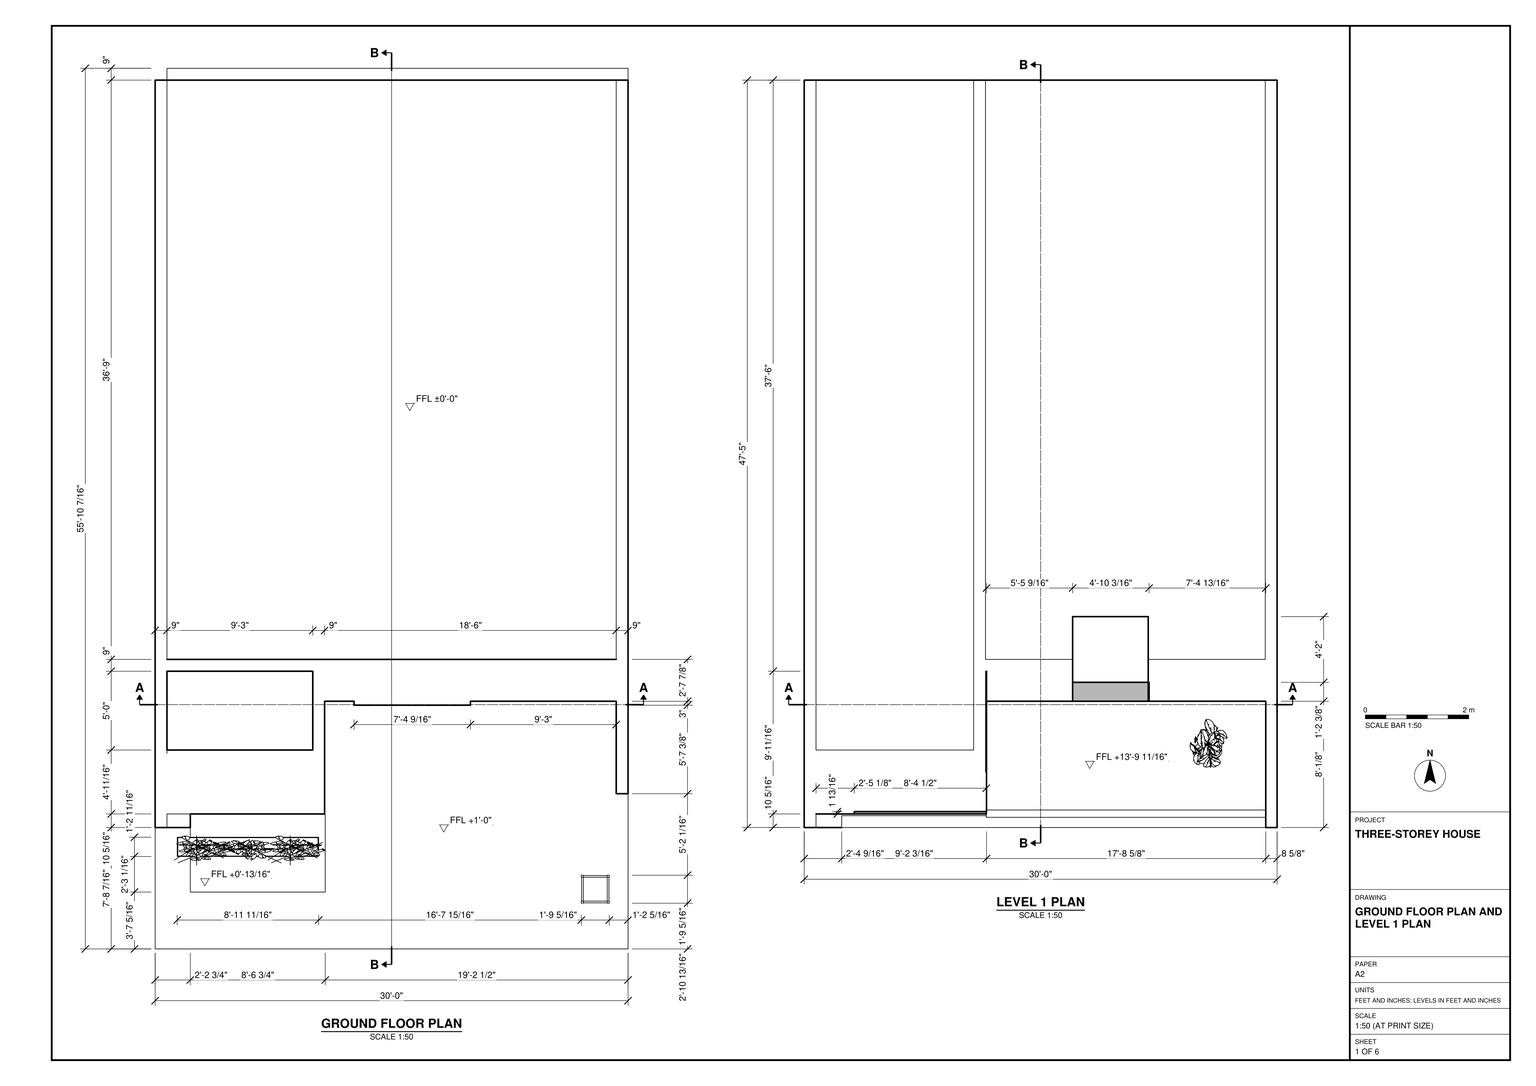
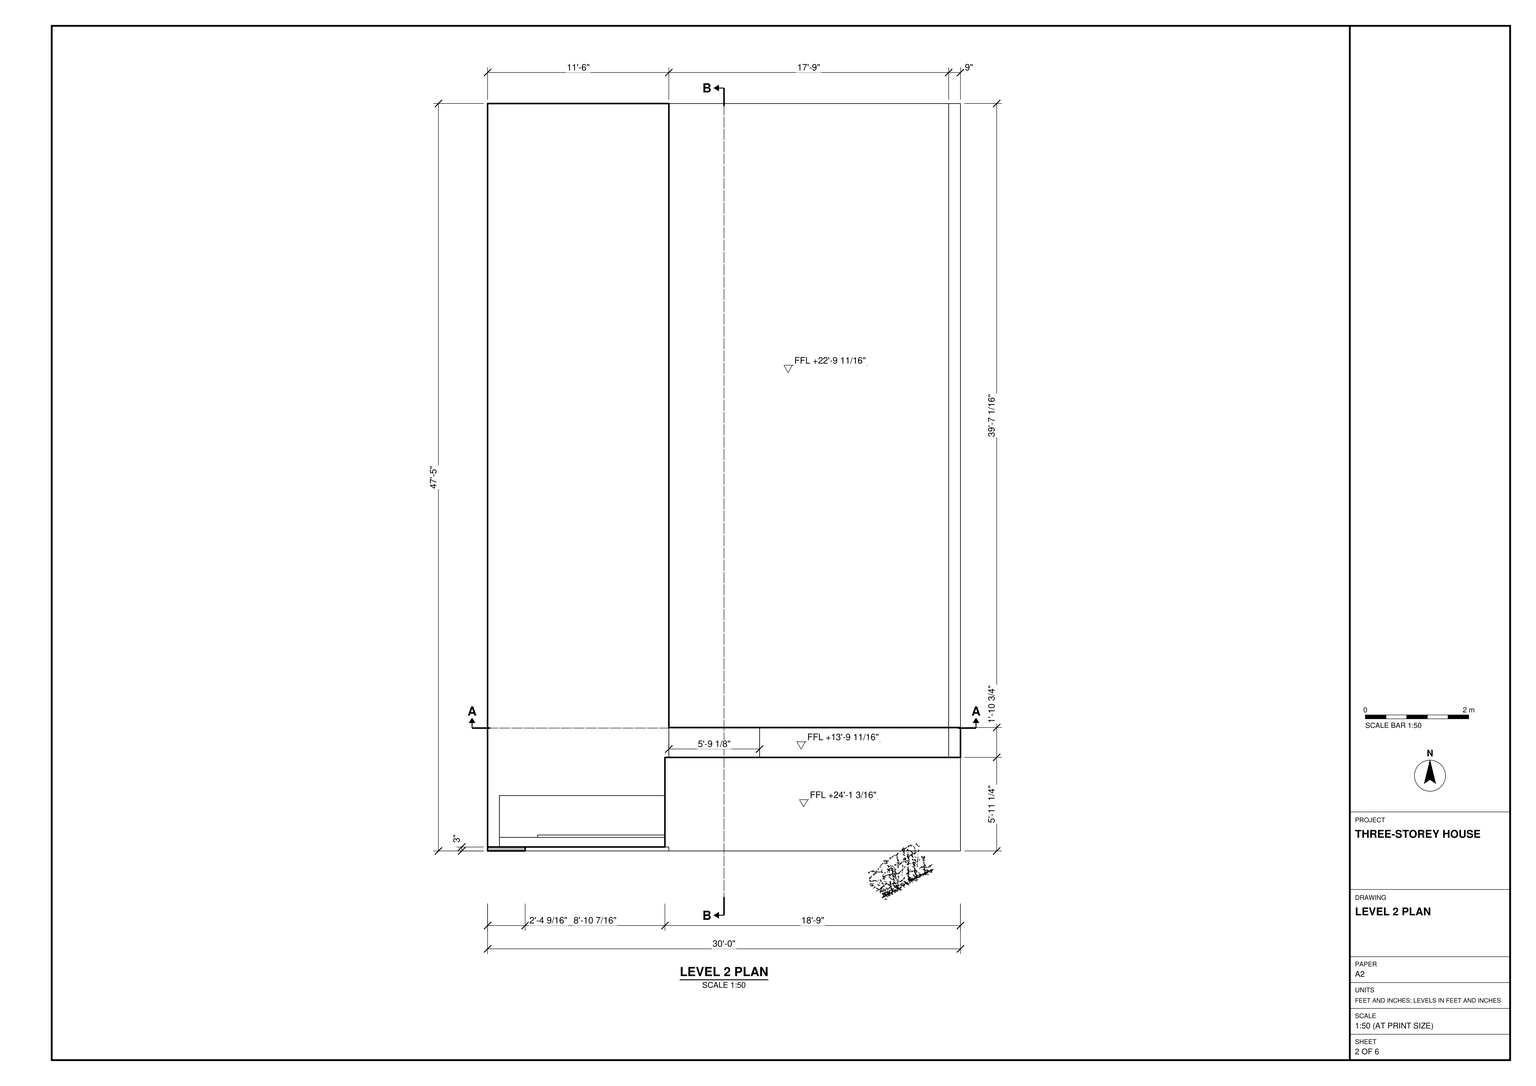
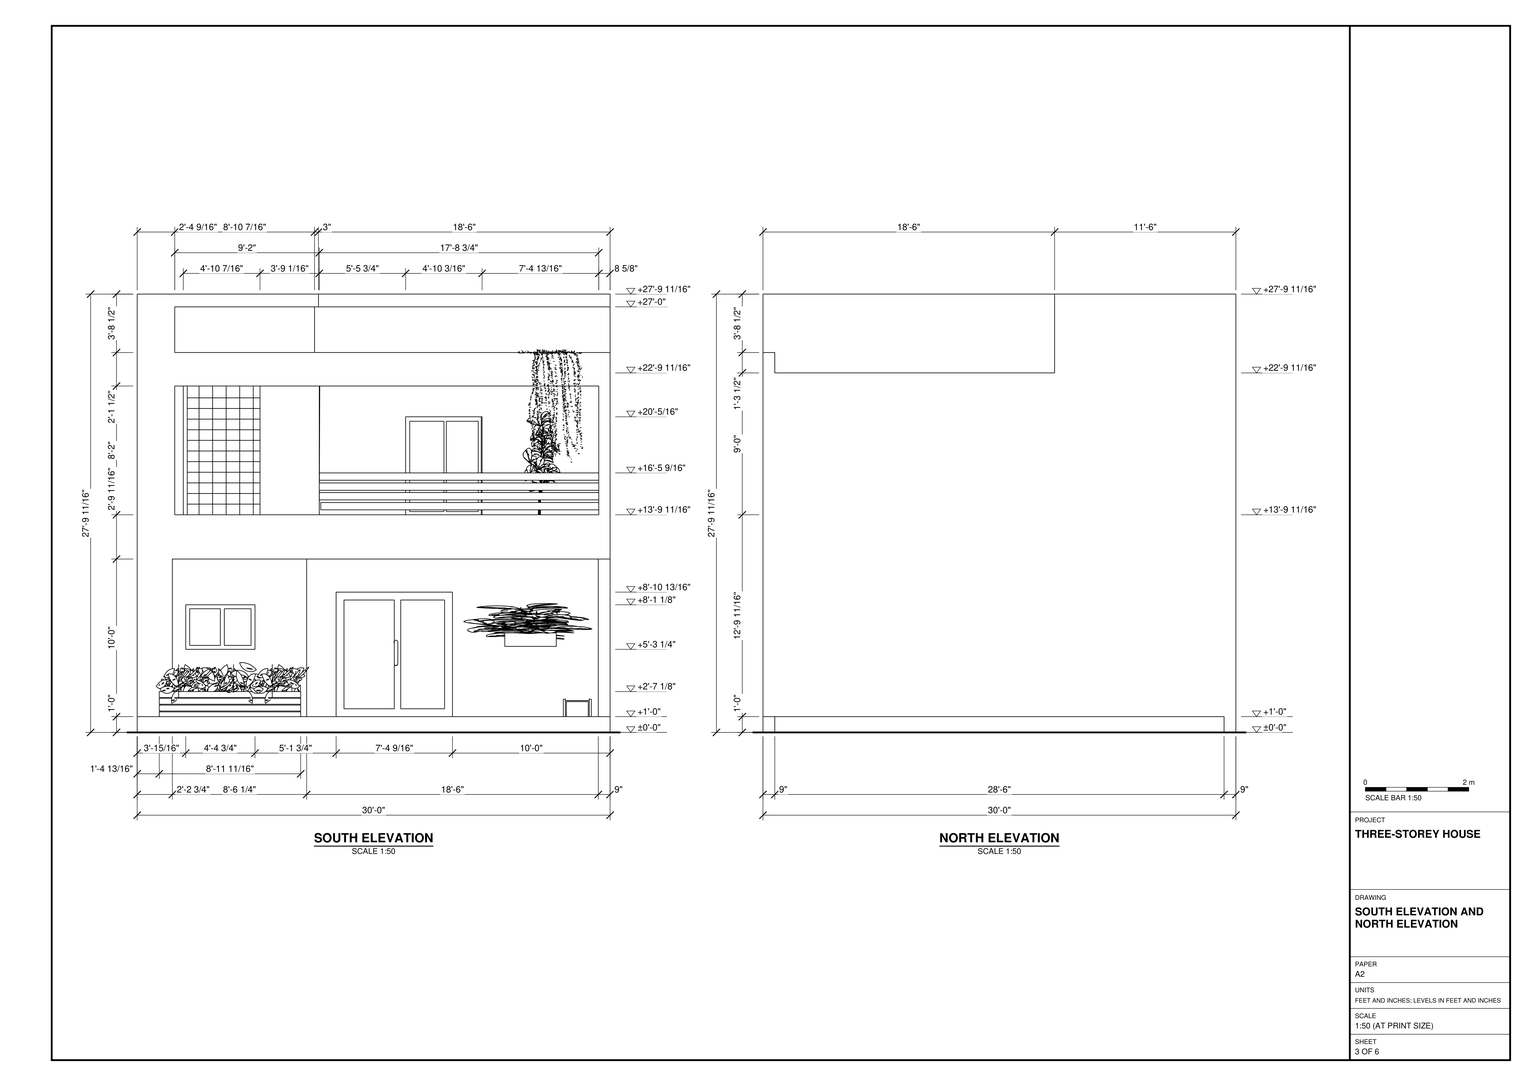
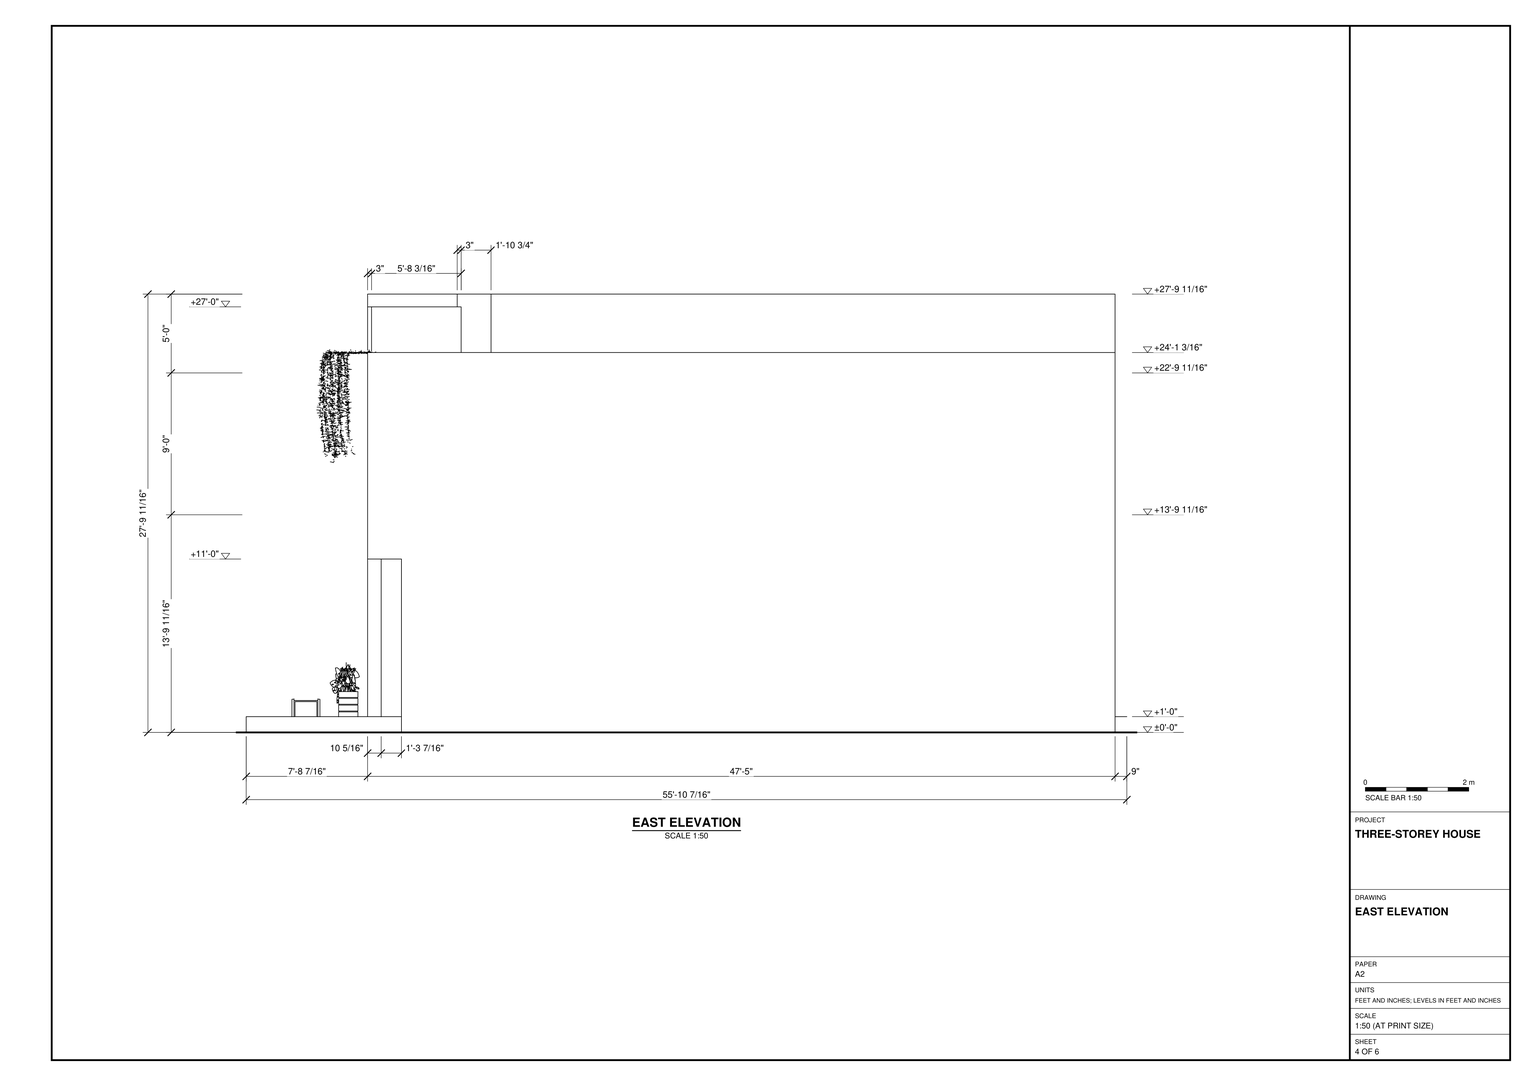
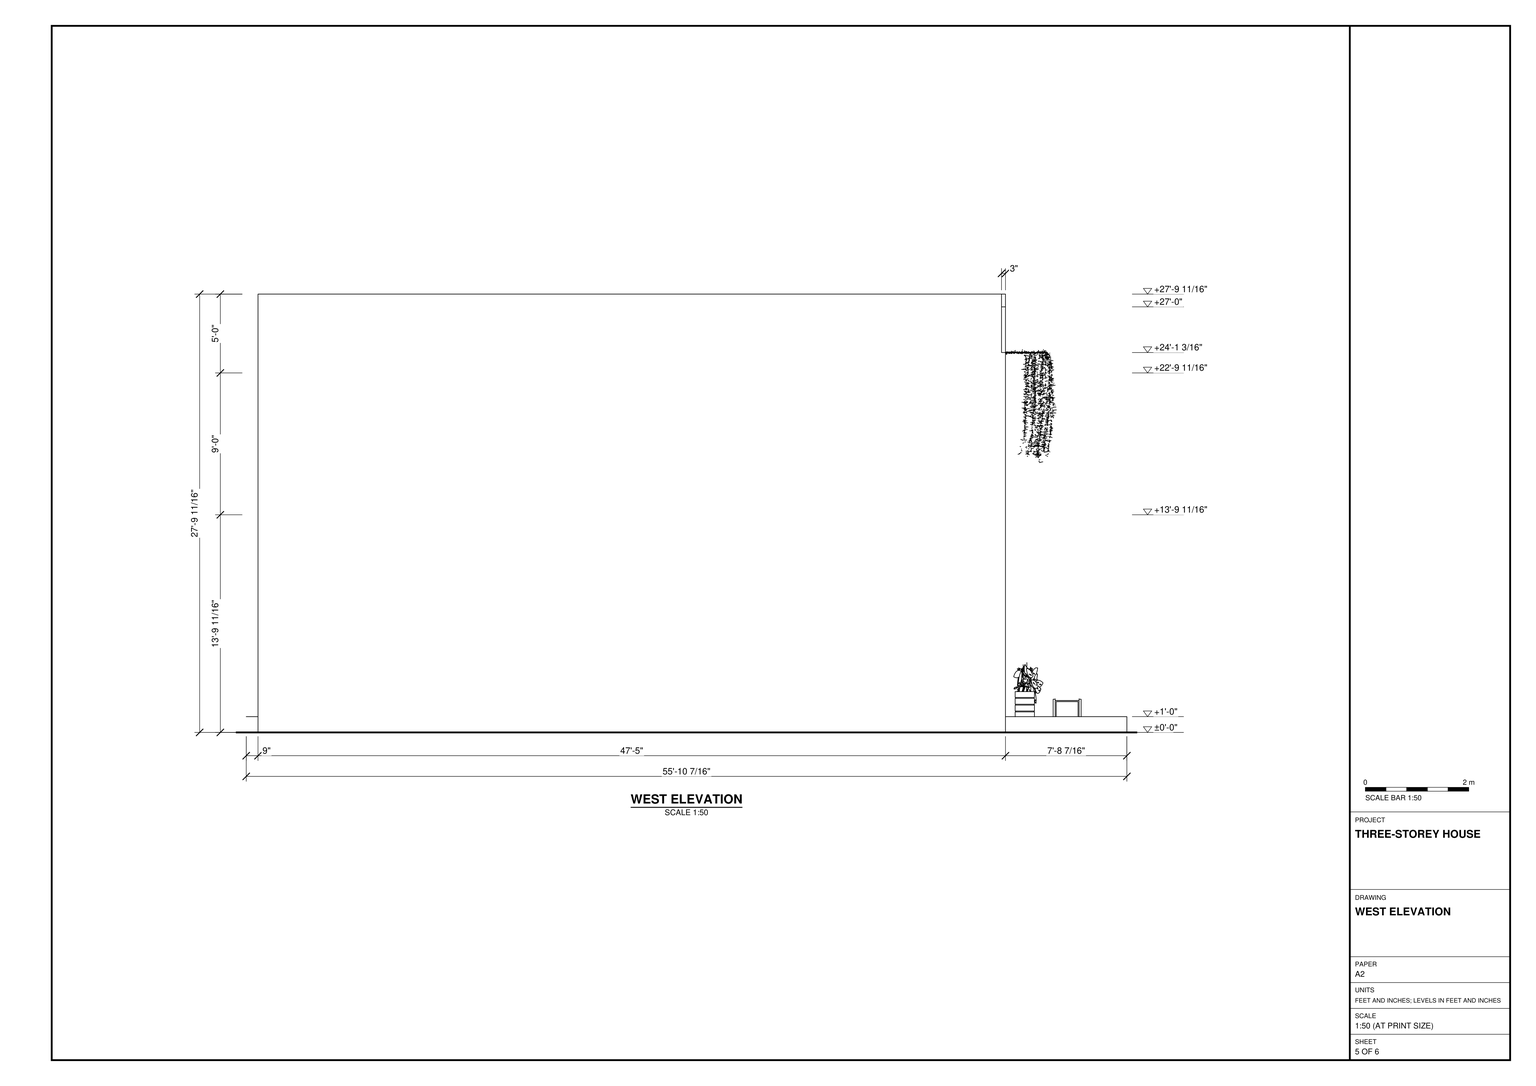
Build the three-storey house shown in task_files/diagram_01.pdf as a SketchUp model. Work in feet and inches. Set the overall width to 30'-0", the front-to-back depth to 55'-10 7/16", and the height to 27'-9 11/16". Use finished floor levels of ±0'-0", +13'-9 11/16", and +22'-9 11/16".

Use the plans to lay out the rectangular base, the stepped ground-floor frontage, the floor slabs, and the walls at their drawn thicknesses, including the 9" perimeter walls. Keep the base extending south beyond the upper floors. On the south elevation, place the paired entrance doors to the right of the smaller window, with the low planted bed beneath the window. Above the entrance, form the recessed balcony with its horizontal railing and paired doors. Model the gridded panel in the adjacent bay. Match the flat roof areas and their changes in height to the upper plan and elevations, including the long horizontal frame above the balcony. Any suitable library components may be used for plants and other loose decor.

Keep walls, slabs, roof elements, and each furniture or joinery piece shown in separate groups or components. Use components for repeated parts. Save one SketchUp model as output_files/three_storey_house_with_a_recessed_south_balcony.skp.

# SketchUp Ruby script. Lengths in inches.
U = 1.inch
M = Sketchup.active_model
def pt(a) = Geom::Point3d.new(a.map { |v| v * U })
def face(e, loops, mat)
  f = e.add_face(loops[0].map { |a| pt(a) })
  loops[1..].each { |l| e.add_face(l.map { |a| pt(a) }).erase! }
  f.material = f.back_material = mat if mat
  f
end
# faces: each face lists its corners as indices into pts; further lists are holes
def faces(e, pts, list, mat = nil) = list.each { |f| face(e, (f[0].is_a?(Array) ? f : [f]).map { |l| l.map { |i| pts[i] } }, mat) }
# xy, xz, yz: faces in a plane at the given z, y or x. An outline is a flat list of corners, or four numbers for a rectangle; further outlines are holes
def ring(l) = l.size == 4 ? [[l[0], l[1]], [l[2], l[1]], [l[2], l[3]], [l[0], l[3]]] : l.each_slice(2).to_a
def flat(e, list, mat, &to3) = list.each { |f| face(e, (f[0].is_a?(Array) ? f : [f]).map { |l| ring(l).map { |u, v| to3.(u, v) } }, mat) }
def xy(e, z, list, mat = nil) = flat(e, list, mat) { |x, y| [x, y, z] }
def xz(e, y, list, mat = nil) = flat(e, list, mat) { |x, z| [x, y, z] }
def yz(e, x, list, mat = nil) = flat(e, list, mat) { |y, z| [x, y, z] }
def lines(e, pts, list) = list.each { |a, b| e.add_line(pt(pts[a]), pt(pts[b])) }
# prism: a flat outline (further loops are holes) pulled along v
def prism(e, loops, v, mat = nil)
  f = face(e, loops, mat); d = Geom::Vector3d.new(v.map { |x| x * U })
  f.pushpull(f.normal.samedirection?(d) ? d.length : -d.length)
end
def box(e, o, s, mat = nil) = prism(e, [[o, [o[0] + s[0], o[1], o[2]], [o[0] + s[0], o[1] + s[1], o[2]], [o[0], o[1] + s[1], o[2]]]], [0, 0, s[2]], mat)
def at(x, y, z, deg = 0) = Geom::Transformation.translation(pt([x, y, z])) * Geom::Transformation.rotation(ORIGIN, Z_AXIS, deg.degrees)
def axes(o, x, y, z) = Geom::Transformation.new([*x, 0, *y, 0, *z, 0, *pt(o).to_a, 1])
def part(name) = M.definitions.add(name)
# library, detail: a bought-in or finely detailed component or shape, given as its bounding box
def library(name, o, s) = part(name).tap { |d| box(d.entities, o, s) }
def detail(e, o, s) = box(e.add_group.entities, o, s)
def put(e, d, t, mat = nil) = e.add_instance(d, t).tap { |i| i.material = mat if mat }
def group(e, t, mat = nil) = e.add_group.tap { |g| g.transformation = t; g.material = mat if mat }.entities
root = M.entities
M.materials.add("!长灌木1").color = [90, 107, 61]
M.materials.add("Brick_14_1K").color = [201, 199, 193]
M.materials.add("Glass_Mirror_01").color = [185, 185, 185]
M.materials.add("Glass_Sky Reflection_01").color = [126, 138, 183]
M.materials["Glass_Sky Reflection_01"].alpha = 0.25
M.materials.add("Material20").color = [184, 138, 65]
M.materials.add("Material48").color = [126, 124, 110]
M.materials.add("Material~1").color = [39, 255, 54]
M.materials.add("Metal_32_1K").color = [117, 124, 125]
M.materials.add("Plywood_08_1K").color = [202, 166, 113]
M.materials.add("ThomThom - Buttons2").color = [40, 40, 43]
M.materials.add("ThomThom - Waistcoat2").color = [127, 127, 126]
M.materials.add("Wood_Floor_01_1K").color = [146, 111, 76]
M.materials.add("Wood_Planks_01_1K").color = [69, 67, 63]
M.materials.add("Wood_Veneer_15_1K").color = [103, 69, 45]
M.materials.add("[Cladding_Siding_Tan]").color = [83, 83, 83]
M.materials.add("avelã ou canyon").color = [164, 137, 111]
c1 = part("Wooden planter box")
xy(c1.entities,0,[[13.83,7.95,28.79,88.09]],"[Cladding_Siding_Tan]")
xy(c1.entities,22.64,[[13.83,7.95,28.79,88.09]],"[Cladding_Siding_Tan]")
xz(c1.entities,7.95,[[13.83,3.9375,28.79,4.53],[13.83,8.46,28.79,9.06],[13.83,12.99,28.79,13.58],[13.83,17.52,28.79,18.11],[13.83,22.05,28.79,22.64]],"[Cladding_Siding_Tan]")
xz(c1.entities,88.09,[[13.83,3.9375,28.79,4.53],[13.83,8.46,28.79,9.06],[13.83,12.99,28.79,13.58],[13.83,17.52,28.79,18.11],[13.83,22.05,28.79,22.64]],"[Cladding_Siding_Tan]")
yz(c1.entities,13.83,[[7.95,3.9375,88.09,4.53],[7.95,8.46,88.09,9.06],[7.95,12.99,88.09,13.58],[7.95,17.52,88.09,18.11],[7.95,22.05,88.09,22.64]],"[Cladding_Siding_Tan]")
yz(c1.entities,28.79,[[7.95,3.9375,88.09,4.53],[7.95,8.46,88.09,9.06],[7.95,12.99,88.09,13.58],[7.95,17.52,88.09,18.11],[7.95,22.05,88.09,22.64]],"[Cladding_Siding_Tan]")
g1 = group(c1.entities,at(13.4375,7.55,0))
prism(g1,[[[15.75,80.93,22.64],[15.75,0,22.64],[0,0,22.64],[0,80.93,22.64]],[[0.39,80.53,22.64],[0.39,0.39,22.64],[15.35,0.39,22.64],[15.35,80.53,22.64]]],[0,0,3.9375],"avelã ou canyon")
prism(g1,[[[15.75,80.93,9.06],[15.75,0,9.06],[0,0,9.06],[0,80.93,9.06]],[[0.39,80.53,9.06],[0.39,0.39,9.06],[15.35,0.39,9.06],[15.35,80.53,9.06]]],[0,0,3.9375],"avelã ou canyon")
prism(g1,[[[15.75,80.93,13.58],[15.75,0,13.58],[0,0,13.58],[0,80.93,13.58]],[[0.39,80.53,13.58],[0.39,0.39,13.58],[15.35,0.39,13.58],[15.35,80.53,13.58]]],[0,0,3.9375],"avelã ou canyon")
prism(g1,[[[15.75,80.93,0],[15.75,0,0],[0,0,0],[0,80.93,0]],[[0.39,80.53,0],[0.39,0.39,0],[15.35,0.39,0],[15.35,80.53,0]]],[0,0,3.9375],"avelã ou canyon")
prism(g1,[[[15.75,80.93,4.53],[15.75,0,4.53],[0,0,4.53],[0,80.93,4.53]],[[0.39,80.53,4.53],[0.39,0.39,4.53],[15.35,0.39,4.53],[15.35,80.53,4.53]]],[0,0,3.9375],"avelã ou canyon")
prism(g1,[[[15.75,80.93,18.11],[15.75,0,18.11],[0,0,18.11],[0,80.93,18.11]],[[0.39,80.53,18.11],[0.39,0.39,18.11],[15.35,0.39,18.11],[15.35,80.53,18.11]]],[0,0,3.9375],"avelã ou canyon")
c2 = library("Bush\#1",[-12.92,-38.23,78.84],[28.51,16.75,15.79])
c3 = library("Bush",[-8.21,-45.67,79.34],[21.65,20.96,14.54])
c4 = library("Group6\#1",[8874.76,-5589.78,-33.6],[50.13,38.07,87.13])
c5 = part("组\#1")
xy(c5.entities,0,[[0,0,2.36,2.36],[29.92,0,32.28,2.36],[0,29.92,2.36,32.28],[29.92,29.92,32.28,32.28]],"Material48")
xy(c5.entities,1.57,[[2.36,0.39,2.36,2.36,0.39,2.36,0.39,29.92,2.36,29.92,2.36,31.89,29.92,31.89,29.92,29.92,31.89,29.92,31.89,2.36,29.92,2.36,29.92,0.39]],"Material48")
xy(c5.entities,2.76,[[3.54,0.39,28.74,1.57],[0.39,3.54,1.57,28.74],[30.71,3.54,31.89,28.74],[3.54,30.71,28.74,31.89]],"Material20")
xy(c5.entities,20.08,[[3.54,0.39,28.74,1.57],[0.39,3.54,1.57,28.74],[30.71,3.54,31.89,28.74],[3.54,30.71,28.74,31.89]],"Material20")
xy(c5.entities,21.0625,[[2.36,2.36,29.92,29.92]],"!长灌木1")
xy(c5.entities,21.26,[[2.36,0.39,29.92,2.36],[0.39,2.36,2.36,29.92],[29.92,2.36,31.89,29.92],[2.36,29.92,29.92,31.89]],"Material20")
xy(c5.entities,21.38,[[2.36,2.36,29.92,29.92]],"!长灌木1")
xy(c5.entities,22.83,[[0,0,2.36,2.36],[29.92,0,32.28,2.36],[0,29.92,2.36,32.28],[29.92,29.92,32.28,32.28]],"Material20")
xz(c5.entities,0,[[0,0,2.36,22.83],[29.92,0,32.28,22.83]],"Material20")
xz(c5.entities,0.39,[[[2.36,1.57,29.92,21.26],[3.54,2.76,28.74,20.08]]],"Material20")
xz(c5.entities,1.57,[[3.54,2.76,28.74,20.08]],"Material20")
xz(c5.entities,2.36,[[2.36,21.0625,29.92,21.38],[2.36,21.26,29.92,23.43]],"!长灌木1")
xz(c5.entities,2.36,[[0,0,0,22.83,2.36,22.83,2.36,21.26,0.39,21.26,0.39,1.57,2.36,1.57,2.36,0],[29.92,0,29.92,1.57,31.89,1.57,31.89,21.26,29.92,21.26,29.92,22.83,32.28,22.83,32.28,0]],"Material20")
xz(c5.entities,3.54,[[0.39,2.76,1.57,20.08],[30.71,2.76,31.89,20.08]],"Material20")
xz(c5.entities,28.74,[[0.39,2.76,1.57,20.08],[30.71,2.76,31.89,20.08]],"Material20")
xz(c5.entities,29.92,[[2.36,21.0625,29.92,21.38],[2.36,21.26,29.92,23.43]],"!长灌木1")
xz(c5.entities,29.92,[[0,0,2.36,0,2.36,1.57,0.39,1.57,0.39,22.83,0,22.83],[29.92,0,32.28,0,32.28,22.83,31.89,22.83,31.89,1.57,29.92,1.57],[0.39,21.26,2.36,22.83],[29.92,21.26,31.89,22.83]],"Material20")
xz(c5.entities,30.71,[[3.54,2.76,28.74,20.08]],"Material20")
xz(c5.entities,31.89,[[[2.36,1.57,29.92,21.26],[3.54,2.76,28.74,20.08]]],"Material20")
xz(c5.entities,32.28,[[0,0,2.36,22.83],[29.92,0,32.28,22.83]],"Material20")
yz(c5.entities,0,[[0,0,2.36,22.83],[29.92,0,32.28,22.83]],"Material20")
yz(c5.entities,0.39,[[[2.36,1.57,29.92,21.26],[3.54,2.76,28.74,20.08]]],"Material20")
yz(c5.entities,1.57,[[3.54,2.76,28.74,20.08]],"Material20")
yz(c5.entities,2.36,[[0,0,2.36,0,2.36,1.57,0.39,1.57,0.39,22.83,0,22.83]])
yz(c5.entities,2.36,[[2.36,21.0625,29.92,21.38],[2.36,21.26,29.92,23.43]],"!长灌木1")
yz(c5.entities,2.36,[[29.92,0,32.28,0,32.28,22.83,29.92,22.83,29.92,21.26,31.89,21.26,31.89,1.57,29.92,1.57],[0.39,21.26,2.36,22.83]],"Material20")
yz(c5.entities,3.54,[[0.39,2.76,1.57,20.08],[30.71,2.76,31.89,20.08]],"Material20")
yz(c5.entities,28.74,[[0.39,2.76,1.57,20.08],[30.71,2.76,31.89,20.08]],"Material20")
yz(c5.entities,29.92,[[2.36,21.0625,29.92,21.38],[2.36,21.26,29.92,23.43]],"!长灌木1")
yz(c5.entities,29.92,[[0,0,0,22.83,2.36,22.83,2.36,21.26,0.39,21.26,0.39,1.57,2.36,1.57,2.36,0],[29.92,0,29.92,1.57,31.89,1.57,31.89,21.26,29.92,21.26,29.92,22.83,32.28,22.83,32.28,0]],"Material20")
yz(c5.entities,30.71,[[3.54,2.76,28.74,20.08]],"Material20")
yz(c5.entities,31.89,[[[2.36,1.57,29.92,21.26],[3.54,2.76,28.74,20.08]]],"Material20")
yz(c5.entities,32.28,[[0,0,2.36,22.83],[29.92,0,32.28,22.83]],"Material20")
c6 = part("组\#2")
put(c6.entities,c5,at(24.1,23.99,0))
c7 = library("Group38\#2",[14.01,28.44,-23.43],[18.58,18.32,38.89])
xy(root,-12,[[0,0,0,92.43,9,92.43,9,102.77,129,102.77,129,142.43,351,142.43,351,118.19,360,118.19,360,0],[[0,92.43,9,92.43,9,102.77,129,102.77,129,188.58,151.43,188.58,151.43,185.58,240,185.58,240,188.58,351,188.58,351,118.19,360,118.19,360,661.43,351,661.43,351,220.43,9,220.43,9,661.43,0,661.43],[9,151.43,120,211.43]],[9,151.43,120,211.43],[9,220.43,351,661.43]])
xy(root,-11.2,[[26.77,43.3,129.49,102.77],[9,92.43,26.77,102.77]])
xy(root,0,[[0,0,360,0,360,118.19,351,118.19,351,188.58,240,188.58,240,185.58,151.43,185.58,151.43,188.58,129,188.58,129,102.77,129.49,102.77,129.49,43.3,26.77,43.3,26.77,92.43,0,92.43],[9,661.43,360,670.43]])
xy(root,51.26,[[36.94,102.77,89.67,188.58]])
xy(root,53.5,[[279.82,154.66,319.02,188.58]],"ThomThom - Waistcoat2")
xy(root,58.53,[[284.25,159.09,314.59,184.15]],"Wood_Veneer_15_1K")
xy(root,63.77,[[[279.82,154.66,319.02,188.58],[284.25,159.09,314.59,184.15]]],"Plywood_08_1K")
xy(root,85.15,[[36.94,102.77,89.67,188.58]])
xy(root,94.8,[[151.43,185.58,240,188.58]])
xy(root,120,[[26.77,92.43,129,102.77],[129,92.43,351,188.58],[351,92.43,360,118.19],[9,151.43,120,211.43]])
xy(root,153.7,[[28.58,92.43,351.38,101.43],[138.6,101.43,351.38,104.56],[38.09,102.77,138.6,104.56],[138,134.6,138.6,211.43],[204.34,188.58,261.9,253]])
xy(root,153.7,[[138.6,104.56,351.38,188.58]],"Glass_Mirror_01")
xy(root,228.29,[[204.34,188.58,261.9,253]],"ThomThom - Waistcoat2")
xy(root,251.7,[[138.98,92.43,138.98,188.58,207.1,188.58,207.1,186.4,351.38,186.4,351.38,92.43],[9,102.77,9,134.6,138.6,134.6,138.6,104.56,38.09,104.56,38.09,102.77],[38.09,102.77,138.6,104.56],[207.1,186.4,351,188.58],[351,186.4,351.38,188.58],
  [138.98,188.58,207.1,211.43]])
xy(root,261.7,[[138,163.64,207.1,186.4],[138,186.4,351,661.43]])
xy(root,277.21,[[28.58,92.43,138,95.43],[138,92.43,360,92.43,360,160.64,351,160.64,351,163.64,135,163.64,135,95.43,138,95.43],[351,160.64,360,163.64],[351,163.64,360,186.4],[351,186.4,360,661.43]])
xy(root,311.98,[[28.58,92.43,138,95.43],[135,95.43,138,163.64],[138,160.64,207.1,163.64],[207.1,160.64,360,163.64]])
xy(root,321.7,[[0,92.43,138,92.43,138,160.64,360,160.64,360,186.4,138,186.4,138,661.43,0,661.43]])
xz(root,0,[[0,-12,360,0]])
xz(root,43.3,[[26.77,-11.2,129.49,0]])
xz(root,92.43,[[[0,0,26.77,0,26.77,120,360,120,360,277.21,28.58,277.21,28.58,311.98,138,311.98,138,321.7,0,321.7],[28.58,153.7,351.38,251.7]]])
xz(root,95.43,[[0,277.21,28.58,311.98],[28.58,277.21,135,311.98]],"ThomThom - Waistcoat2")
xz(root,102.77,[[129,-11.2,129.49,0]])
xz(root,102.77,[[9,-12,129,-11.2],[[26.77,-11.2,129,120],[36.94,51.26,89.67,85.15]]],"Brick_14_1K")
xz(root,102.77,[[39.94,54.26,63.3,82.15],[66.3,54.26,86.67,82.15]],"Glass_Mirror_01")
xz(root,102.77,[[38.09,153.7,47.09,161.79],[47.09,153.7,57.41,161.79],[57.41,153.7,67.72,161.79],[67.72,153.7,78.04,161.79],[78.04,153.7,88.35,161.79],
  [88.35,153.7,93.51,161.79],[38.09,161.79,47.09,169.88],[47.09,161.79,57.41,169.88],[57.41,161.79,67.72,169.88],[67.72,161.79,78.04,169.88],
  [78.04,161.79,88.35,169.88],[88.35,161.79,93.51,169.88],[38.09,169.88,47.09,177.97],[47.09,169.88,57.41,177.97],[57.41,169.88,67.72,177.97],
  [67.72,169.88,78.04,177.97],[78.04,169.88,88.35,177.97],[88.35,169.88,93.51,177.97],[38.09,177.97,47.09,186.06],[47.09,177.97,57.41,186.06],
  [57.41,177.97,67.72,186.06],[67.72,177.97,78.04,186.06],[78.04,177.97,88.35,186.06],[88.35,177.97,93.51,186.06],[38.09,186.06,47.09,194.16],
  [47.09,186.06,57.41,194.16],[57.41,186.06,67.72,194.16],[67.72,186.06,78.04,194.16],[78.04,186.06,88.35,194.16],[88.35,186.06,93.51,194.16],
  [38.09,194.16,47.09,202.25],[47.09,194.16,57.41,202.25],[57.41,194.16,67.72,202.25],[67.72,194.16,78.04,202.25],[78.04,194.16,88.35,202.25],
  [88.35,194.16,93.51,202.25],[38.09,202.25,47.09,210.34],[47.09,202.25,57.41,210.34],[57.41,202.25,67.72,210.34],[67.72,202.25,78.04,210.34],
  [78.04,202.25,88.35,210.34],[88.35,202.25,93.51,210.34],[38.09,210.34,47.09,218.43],[47.09,210.34,57.41,218.43],[57.41,210.34,67.72,218.43],
  [67.72,210.34,78.04,218.43],[78.04,210.34,88.35,218.43],[88.35,210.34,93.51,218.43],[38.09,218.43,47.09,226.52],[47.09,218.43,57.41,226.52],
  [57.41,218.43,67.72,226.52],[67.72,218.43,78.04,226.52],[78.04,218.43,88.35,226.52],[88.35,218.43,93.51,226.52],[38.09,226.52,47.09,234.61],
  [47.09,226.52,57.41,234.61],[57.41,226.52,67.72,234.61],[67.72,226.52,78.04,234.61],[78.04,226.52,88.35,234.61],[88.35,226.52,93.51,234.61],
  [38.09,234.61,47.09,242.7],[47.09,234.61,57.41,242.7],[57.41,234.61,67.72,242.7],[67.72,234.61,78.04,242.7],[78.04,234.61,88.35,242.7],
  [88.35,234.61,93.51,242.7],[38.09,242.7,47.09,251.7],[47.09,242.7,57.41,251.7],[57.41,242.7,67.72,251.7],[67.72,242.7,78.04,251.7],
  [78.04,242.7,88.35,251.7],[88.35,242.7,93.51,251.7]],"Glass_Sky Reflection_01")
xz(root,102.77,[[[36.94,51.26,89.67,85.15],[39.94,54.26,63.3,82.15],[66.3,54.26,86.67,82.15]],[35.09,153.7,38.09,251.7]],"Metal_32_1K")
xz(root,102.77,[[9,153.7,35.09,251.7],[93.51,153.7,138.6,251.7]],"ThomThom - Waistcoat2")
xz(root,104.56,[[38.09,153.7,138.6,251.7],[138.6,153.7,138.61,155.56,138.61,157.58,138.98,251.7,138.6,251.7]],"ThomThom - Waistcoat2")
xz(root,118.19,[[351,-12,360,0],[351,0,360,120]])
xz(root,151.43,[[9,-12,120,120]])
xz(root,154.66,[[279.82,53.5,319.02,63.77]],"Plywood_08_1K")
xz(root,159.09,[[284.25,58.53,314.59,63.77]],"ThomThom - Waistcoat2")
xz(root,160.64,[[138,311.98,360,321.7]])
xz(root,163.64,[[138,261.7,207.1,277.21]])
xz(root,163.64,[[135,277.21,360,311.98]],"ThomThom - Waistcoat2")
xz(root,169.96,[[196.91,55.24,196.52,55.29,196.16,55.4375,195.86,55.67,195.71,55.86,195.71,57.59,195.86,57.77,196.16,58.01,196.52,58.16,196.91,58.21,197.29,58.16,197.65,58.01,197.96,57.77,198.19,57.46,198.34,57.11,198.39,56.72,198.34,56.34,198.19,55.98,197.96,55.67,197.65,55.4375,197.29,55.29]],"Wood_Floor_01_1K")
xz(root,170.0625,[[196.91,38.8125,197.29,38.86,197.65,39.01,197.96,39.25,198.19,39.55,198.34,39.91,198.39,40.3,198.38,40.39,198.34,40.1,198.19,39.74,197.96,39.43,197.65,39.2,197.29,39.05,196.91,39,196.52,39.05,196.16,39.2,195.86,39.43,195.71,39.62,195.71,39.43,195.86,39.25,196.16,39.01,196.52,38.86]],"Wood_Floor_01_1K")
xz(root,184.15,[[284.25,58.53,314.59,63.77]],"Wood_Veneer_15_1K")
xz(root,185.58,[[151.43,-12,240,0]])
xz(root,185.58,[[157.43,6,195.71,6,195.71,55.86,195.62,55.98,195.47,56.34,195.42,56.72,195.47,57.11,195.62,57.46,195.71,57.59,195.71,88.8,157.43,88.8],[200.62,6,234,88.8],[195.71,55.86,195.71,57.59,195.62,57.46,195.47,57.11,195.42,56.72,195.47,56.34,195.62,55.98]],"Glass_Mirror_01")
xz(root,185.58,[[[151.43,0,240,94.8],[157.43,6,157.43,88.8,195.71,88.8,195.71,57.59,195.86,57.77,196.16,58.01,196.52,58.16,196.91,58.21,197.29,58.16,197.65,58.01,197.96,57.77,198.19,57.46,198.34,57.11,198.39,56.72,198.34,56.34,198.19,55.98,197.96,55.67,197.65,55.4375,197.29,55.29,196.91,55.24,196.52,55.29,196.16,55.4375,195.86,55.67,195.71,55.86,195.71,41.16,195.86,41.35,196.16,41.58,196.52,41.73,196.91,41.78,197.29,41.73,197.65,41.58,197.96,41.35,198.19,41.04,198.34,40.68,198.39,40.3,198.34,39.91,198.19,39.55,197.96,39.25,197.65,39.01,197.29,38.86,196.91,38.8125,196.52,38.86,196.16,39.01,195.86,39.25,195.71,39.43,195.71,6],[200.62,6,234,88.8]]],"Wood_Floor_01_1K")
xz(root,186.4,[[207.1,251.7,351,261.7],[138,261.7,138,321.7,360,321.7,360,277.21,351,277.21,351,261.7]])
xz(root,188.58,[[129,-12,151.43,0],[240,-12,351,0],[36.94,51.26,89.67,85.15]])
xz(root,188.58,[[[129,0,151.43,0,151.43,94.8,240,94.8,240,0,351,0,351,120,129,120],[279.82,53.5,319.02,63.77]],[138.6,153.7,204.34,153.7,204.34,228.29,261.9,228.29,261.9,153.7,351.38,153.7,351.38,251.7,138.98,251.7]],"ThomThom - Waistcoat2")
xz(root,211.43,[[9,-12,120,120]])
xz(root,220.43,[[9,-12,351,120]])
xz(root,253,[[204.34,153.7,261.9,228.29]],"ThomThom - Waistcoat2")
xz(root,661.43,[[0,-12,0,321.7,138,321.7,138,261.7,351,261.7,351,277.21,360,277.21,360,0,9,0,9,-12],[9,-12,351,0],[351,-12,360,0]])
yz(root,0,[[0,-12,92.43,0],[92.43,-12,92.43,277.21,95.43,277.21,95.43,321.7,661.43,321.7,661.43,-12],[92.43,277.21,95.43,311.98],[92.43,311.98,95.43,321.7]])
yz(root,9,[[92.43,-12,102.77,-11.2],[151.43,-12,211.43,120]])
yz(root,26.77,[[43.3,-11.2,102.77,-11.2,102.77,120,92.43,120,92.43,0,43.3,0]])
yz(root,28.58,[[92.43,277.21,95.43,311.98]])
yz(root,36.94,[[102.77,51.26,188.58,85.15]])
yz(root,38.09,[[102.77,153.7,104.56,161.79],[102.77,161.79,104.56,169.88],[102.77,169.88,104.56,177.97],[102.77,177.97,104.56,186.06],[102.77,186.06,104.56,194.16],
  [102.77,194.16,104.56,202.25],[102.77,202.25,104.56,210.34],[102.77,210.34,104.56,218.43],[102.77,218.43,104.56,226.52],[102.77,226.52,104.56,234.61],
  [102.77,234.61,104.56,242.7],[102.77,242.7,104.56,251.7]])
yz(root,89.67,[[102.77,51.26,188.58,85.15]])
yz(root,120,[[151.43,-12,211.43,120]])
yz(root,129,[[142.43,-12,188.58,0]])
yz(root,129,[[102.77,-12,142.43,0],[102.77,0,188.58,120]],"ThomThom - Waistcoat2")
yz(root,129.49,[[43.3,-11.2,102.77,0]])
yz(root,135,[[95.43,277.21,163.64,311.98]])
yz(root,138,[[163.64,261.7,186.4,277.21],[186.4,261.7,661.43,321.7],[92.43,311.98,160.64,321.7]])
yz(root,138.6,[[102.77,172.36,102.28,172.43,101.6,172.71,101.03,173.15,100.59,173.73,100.31,174.4,100.21,175.12,100.31,175.84,100.59,176.51,101.03,177.09,101.6,177.53,102.28,177.81,102.77,177.875],[104.56,172.84,104.56,177.4,104.97,177.09,105.41,176.51,105.6875,175.84,105.78,175.12,105.6875,174.4,105.41,173.73,104.97,173.15]])
yz(root,138.6,[[102.77,153.7,102.77,172.36,103,172.33,103.72,172.43,104.39,172.71,104.56,172.84,104.56,153.7],[103,172.33,102.77,172.36,102.77,177.875,103,177.9,103.72,177.81,104.39,177.53,104.56,177.4,104.56,172.84,104.39,172.71,103.72,172.43],[104.56,177.4,104.39,177.53,103.72,177.81,103,177.9,102.77,177.875,102.77,251.7,104.56,251.7]],"ThomThom - Waistcoat2")
yz(root,138.61,[[104.56,155.56,104.56,157.58,104.3,157.54,104.06,157.44,103.85,157.28,103.6875,157.07,103.58,156.83,103.55,156.57,103.58,156.31,103.6875,156.0625,103.85,155.85,104.06,155.69,104.3,155.59]])
yz(root,138.61,[[104.56,155.56,104.82,155.59,105.07,155.69,105.27,155.85,105.44,156.0625,105.54,156.31,105.57,156.57,105.54,156.83,105.44,157.07,105.27,157.28,105.07,157.44,104.82,157.54,104.56,157.58]],"ThomThom - Waistcoat2")
yz(root,138.66,[[103,165.04,102.28,165.13,101.6,165.41,101.03,165.85,100.59,166.43,100.31,167.1,100.21,167.82,100.31,168.54,100.59,169.21,101.03,169.79,101.6,170.23,102.28,170.51,103,170.61,103.72,170.51,104.39,170.23,104.97,169.79,105.41,169.21,105.6875,168.54,105.78,167.82,105.6875,167.1,105.41,166.43,104.97,165.85,104.39,165.41,103.72,165.13],[103,179.98,102.28,180.08,101.6,180.36,101.03,180.8,100.59,181.375,100.31,182.05,100.21,182.77,100.31,183.49,100.59,184.16,101.03,184.74,101.6,185.18,102.28,185.46,103,185.55,103.72,185.46,104.39,185.18,104.97,184.74,105.41,184.16,105.6875,183.49,105.78,182.77,105.6875,182.05,105.41,181.375,104.97,180.8,104.39,180.36,103.72,180.08]])
yz(root,139.74,[[103,157.45,102.28,157.54,101.6,157.82,101.03,158.26,100.59,158.84,100.31,159.51,100.21,160.23,100.31,160.95,100.59,161.625,101.03,162.2,101.6,162.64,102.28,162.92,103,163.02,103.72,162.92,104.39,162.64,104.97,162.2,105.41,161.625,105.6875,160.95,105.78,160.23,105.6875,159.51,105.41,158.84,104.97,158.26,104.39,157.82,103.72,157.54]])
yz(root,151.43,[[185.58,-12,188.58,0],[185.58,0,188.58,94.8]])
yz(root,195.71,[[170.0625,39.43,185.58,41.16],[167.2,39.62,167.2,57.59,169.96,57.59,169.96,55.86,168.93,55.86,168.93,41.35,170.0625,41.35,170.0625,39.62],[169.96,55.86,185.58,57.59]],"Wood_Planks_01_1K")
yz(root,204.34,[[188.58,153.7,253,228.29]],"ThomThom - Waistcoat2")
yz(root,240,[[185.58,-12,188.58,0],[185.58,0,188.58,94.8]])
yz(root,261.9,[[188.58,153.7,253,228.29]],"ThomThom - Waistcoat2")
yz(root,279.82,[[154.66,53.5,188.58,63.77]],"Plywood_08_1K")
yz(root,284.25,[[159.09,58.53,184.15,63.77]],"ThomThom - Waistcoat2")
yz(root,314.59,[[159.09,58.53,184.15,63.77]],"Wood_Veneer_15_1K")
yz(root,319.02,[[154.66,53.5,188.58,63.77]],"ThomThom - Waistcoat2")
yz(root,351,[[118.19,-12,142.43,0],[142.43,-12,188.58,0],[118.19,0,188.58,120],[186.4,251.7,211.43,261.7],[186.4,261.7,661.43,277.21]])
yz(root,351.38,[[[92.43,153.7,188.58,251.7],[103,179.98,103.72,180.08,104.39,180.36,104.97,180.8,105.41,181.375,105.6875,182.05,105.78,182.77,105.6875,183.49,105.41,184.16,104.97,184.74,104.39,185.18,103.72,185.46,103,185.55,102.28,185.46,101.6,185.18,101.03,184.74,100.59,184.16,100.31,183.49,100.21,182.77,100.31,182.05,100.59,181.375,101.03,180.8,101.6,180.36,102.28,180.08],[103,157.45,103.72,157.54,104.39,157.82,104.97,158.26,105.41,158.84,105.6875,159.51,105.78,160.23,105.6875,160.95,105.41,161.625,104.97,162.2,104.39,162.64,103.72,162.92,103,163.02,102.28,162.92,101.6,162.64,101.03,162.2,100.59,161.625,100.31,160.95,100.21,160.23,100.31,159.51,100.59,158.84,101.03,158.26,101.6,157.82,102.28,157.54],[103,165.04,103.72,165.13,104.39,165.41,104.97,165.85,105.41,166.43,105.6875,167.1,105.78,167.82,105.6875,168.54,105.41,169.21,104.97,169.79,104.39,170.23,103.72,170.51,103,170.61,102.28,170.51,101.6,170.23,101.03,169.79,100.59,169.21,100.31,168.54,100.21,167.82,100.31,167.1,100.59,166.43,101.03,165.85,101.6,165.41,102.28,165.13],[103,172.33,103.72,172.43,104.39,172.71,104.97,173.15,105.41,173.73,105.6875,174.4,105.78,175.12,105.6875,175.84,105.41,176.51,104.97,177.09,104.39,177.53,103.72,177.81,103,177.9,102.28,177.81,101.6,177.53,101.03,177.09,100.59,176.51,100.31,175.84,100.21,175.12,100.31,174.4,100.59,173.73,101.03,173.15,101.6,172.71,102.28,172.43]]])
yz(root,360,[[0,-12,118.19,0],[118.19,-12,661.43,-12,661.43,277.21,92.43,277.21,92.43,120,118.19,120],[163.64,277.21,186.4,277.21,186.4,321.7,160.64,321.7,160.64,311.98,163.64,311.98]])
# 35 loose lines left out
p = [[196.52,185.58,38.86],[196.91,185.58,38.8125],[196.91,170.0625,38.8125],[196.52,170.0625,38.86],[197.29,185.58,38.86],[197.29,170.0625,38.86],
  [196.16,185.58,39.01],[196.16,170.0625,39.01],[197.65,185.58,39.01],[197.65,170.0625,39.01],[196.91,166.58,58.21],[196.52,166.63,58.16],
  [196.52,166.63,39.05],[196.91,166.58,39],[196.52,170.0625,39.05],[196.91,170.0625,39],[197.29,166.63,58.16],[197.29,166.63,39.05],
  [197.29,170.0625,39.05],[195.86,185.58,39.25],[195.86,170.0625,39.25],[197.96,185.58,39.25],[197.96,170.0625,39.25],[196.16,166.78,58.01],
  [196.16,166.78,39.2],[196.16,170.0625,39.2],[197.65,166.78,58.01],[197.65,166.78,39.2],[197.65,170.0625,39.2],[195.86,167.01,57.77],
  [195.86,167.01,39.43],[195.86,170.0625,39.43],[197.96,167.01,57.77],[197.96,167.01,39.43],[197.96,170.0625,39.43],[195.71,185.58,39.43],
  [195.71,170.0625,39.43],[198.19,185.58,39.55],[198.19,170.0625,39.55],[195.71,167.2,57.59],[195.71,167.2,39.62],[195.71,170.0625,39.62],
  [198.19,167.32,57.46],[198.19,167.32,39.74],[198.19,170.0625,39.74],[198.34,185.58,39.91],[198.34,170.0625,39.91],[198.34,167.68,57.11],
  [198.34,167.68,40.1],[198.34,170.0625,40.1],[198.39,185.58,40.3],[198.39,170.0625,40.3],[198.39,168.0625,56.72],[198.39,168.0625,40.48],
  [198.38,170.0625,40.39],[198.39,170.0625,40.48],[198.34,185.58,40.68],[198.34,170.0625,40.68],[198.34,168.45,56.34],[198.34,168.45,40.87],
  [198.34,170.0625,40.87],[198.19,185.58,41.04],[198.19,170.0625,41.04],[198.19,168.8,55.98],[198.19,168.8,41.23],[198.19,170.0625,41.23],
  [197.96,185.58,41.35],[197.96,170.0625,41.35],[197.96,169.11,55.67],[197.96,169.11,41.53],[197.96,170.0625,41.53],[195.86,185.58,41.35],
  [195.71,185.58,41.16],[195.71,170.0625,41.16],[195.86,170.0625,41.35],[195.71,168.93,55.86],[195.86,169.11,55.67],[195.86,169.11,41.53],
  [195.71,168.93,41.35],[195.86,170.0625,41.53],[195.71,170.0625,41.35],[196.16,185.58,41.58],[196.16,170.0625,41.58],[197.65,185.58,41.58],
  [197.65,170.0625,41.58],[196.16,169.35,55.4375],[196.16,169.35,41.77],[196.16,170.0625,41.77],[197.65,169.35,55.4375],[197.65,169.35,41.77],
  [197.65,170.0625,41.77],[196.52,185.58,41.73],[196.52,170.0625,41.73],[197.29,185.58,41.73],[197.29,170.0625,41.73],[196.91,185.58,41.78],
  [196.91,170.0625,41.78],[196.52,169.5,55.29],[196.52,169.5,41.92],[196.52,170.0625,41.92],[197.29,169.5,55.29],[197.29,169.5,41.92],
  [197.29,170.0625,41.92],[196.91,169.55,55.24],[196.91,169.55,41.97],[196.91,170.0625,41.97],[196.52,169.96,55.29],[196.91,169.96,55.24],
  [197.29,169.96,55.29],[196.52,185.58,55.29],[196.91,185.58,55.24],[197.29,185.58,55.29],[196.16,169.96,55.4375],[197.65,169.96,55.4375],
  [196.16,185.58,55.4375],[197.65,185.58,55.4375],[195.86,169.96,55.67],[197.96,169.96,55.67],[195.86,185.58,55.67],[197.96,185.58,55.67],
  [198.19,169.96,55.98],[195.71,169.96,55.86],[195.71,185.58,55.86],[198.19,185.58,55.98],[198.34,169.96,56.34],[198.34,185.58,56.34],
  [198.39,169.96,56.72],[198.39,185.58,56.72],[198.34,169.96,57.11],[198.34,185.58,57.11],[198.19,169.96,57.46],[198.19,185.58,57.46],
  [197.96,169.96,57.77],[197.96,185.58,57.77],[195.86,169.96,57.77],[195.71,169.96,57.59],[195.86,185.58,57.77],[195.71,185.58,57.59],
  [196.16,169.96,58.01],[197.65,169.96,58.01],[196.16,185.58,58.01],[197.65,185.58,58.01],[196.52,169.96,58.16],[197.29,169.96,58.16],
  [196.52,185.58,58.16],[197.29,185.58,58.16],[196.91,169.96,58.21],[196.91,185.58,58.21],[138.98,104.56,251.7],[138.61,104.56,157.58],
  [138.61,104.82,157.54],[138.61,105.07,157.44],[138.61,105.27,157.28],[138.61,105.44,157.07],[138.61,105.54,156.83],[138.61,105.57,156.57],
  [138.61,105.54,156.31],[138.61,105.44,156.0625],[138.61,105.27,155.85],[138.61,105.07,155.69],[138.61,104.82,155.59],[138.61,104.56,155.56],
  [138.6,104.56,153.7],[138.6,134.6,153.7],[138.6,188.58,153.7],[138.98,188.58,251.7],[138.6,211.43,153.7],[138.98,211.43,251.7],
  [139.74,103,157.45],[351.38,103,157.45],[351.38,102.28,157.54],[139.74,102.28,157.54],[139.74,103.72,157.54],[351.38,103.72,157.54],
  [351.38,101.6,157.82],[139.74,101.6,157.82],[139.74,104.39,157.82],[351.38,104.39,157.82],[351.38,101.03,158.26],[139.74,101.03,158.26],
  [139.74,104.97,158.26],[351.38,104.97,158.26],[351.38,100.59,158.84],[139.74,100.59,158.84],[139.74,105.41,158.84],[351.38,105.41,158.84],
  [351.38,100.31,159.51],[139.74,100.31,159.51],[139.74,105.6875,159.51],[351.38,105.6875,159.51],[351.38,100.21,160.23],[139.74,100.21,160.23],
  [139.74,105.78,160.23],[351.38,105.78,160.23],[351.38,100.31,160.95],[139.74,100.31,160.95],[139.74,105.6875,160.95],[351.38,105.6875,160.95],
  [351.38,100.59,161.625],[139.74,100.59,161.625],[139.74,105.41,161.625],[351.38,105.41,161.625],[351.38,101.03,162.2],[139.74,101.03,162.2],
  [139.74,104.97,162.2],[351.38,104.97,162.2],[351.38,101.6,162.64],[139.74,101.6,162.64],[139.74,104.39,162.64],[351.38,104.39,162.64],
  [351.38,102.28,162.92],[139.74,102.28,162.92],[139.74,103.72,162.92],[351.38,103.72,162.92],[351.38,103,163.02],[139.74,103,163.02],
  [138.66,103,165.04],[351.38,103,165.04],[351.38,102.28,165.13],[138.66,102.28,165.13],[138.66,103.72,165.13],[351.38,103.72,165.13],
  [351.38,101.6,165.41],[138.66,101.6,165.41],[138.66,104.39,165.41],[351.38,104.39,165.41],[351.38,101.03,165.85],[138.66,101.03,165.85],
  [138.66,104.97,165.85],[351.38,104.97,165.85],[351.38,100.59,166.43],[138.66,100.59,166.43],[138.66,105.41,166.43],[351.38,105.41,166.43],
  [351.38,100.31,167.1],[138.66,100.31,167.1],[138.66,105.6875,167.1],[351.38,105.6875,167.1],[351.38,100.21,167.82],[138.66,100.21,167.82],
  [138.66,105.78,167.82],[351.38,105.78,167.82],[351.38,100.31,168.54],[138.66,100.31,168.54],[138.66,105.6875,168.54],[351.38,105.6875,168.54],
  [351.38,100.59,169.21],[138.66,100.59,169.21],[138.66,105.41,169.21],[351.38,105.41,169.21],[351.38,101.03,169.79],[138.66,101.03,169.79],
  [138.66,104.97,169.79],[351.38,104.97,169.79],[351.38,101.6,170.23],[138.66,101.6,170.23],[138.66,104.39,170.23],[351.38,104.39,170.23],
  [351.38,102.28,170.51],[138.66,102.28,170.51],[138.66,103.72,170.51],[351.38,103.72,170.51],[351.38,103,170.61],[138.66,103,170.61],
  [138.6,102.28,172.43],[138.6,102.77,172.36],[138.6,103,172.33],[351.38,103,172.33],[351.38,102.28,172.43],[138.6,103.72,172.43],
  [351.38,103.72,172.43],[138.6,101.6,172.71],[351.38,101.6,172.71],[138.6,104.39,172.71],[351.38,104.39,172.71],[138.6,101.03,173.15],
  [351.38,101.03,173.15],[138.6,104.56,172.84],[138.6,104.97,173.15],[351.38,104.97,173.15],[138.6,100.59,173.73],[351.38,100.59,173.73],
  [138.6,105.41,173.73],[351.38,105.41,173.73],[138.6,100.31,174.4],[351.38,100.31,174.4],[138.6,105.6875,174.4],[351.38,105.6875,174.4],
  [138.6,100.21,175.12],[351.38,100.21,175.12],[138.6,105.78,175.12],[351.38,105.78,175.12],[138.6,100.31,175.84],[351.38,100.31,175.84],
  [138.6,105.6875,175.84],[351.38,105.6875,175.84],[138.6,100.59,176.51],[351.38,100.59,176.51],[138.6,105.41,176.51],[351.38,105.41,176.51],
  [138.6,101.03,177.09],[351.38,101.03,177.09],[138.6,104.97,177.09],[351.38,104.97,177.09],[138.6,101.6,177.53],[351.38,101.6,177.53],
  [138.6,104.56,177.4],[138.6,104.39,177.53],[351.38,104.39,177.53],[138.6,102.28,177.81],[351.38,102.28,177.81],[138.6,103.72,177.81],
  [351.38,103.72,177.81],[138.6,103,177.9],[138.6,102.77,177.875],[351.38,103,177.9],[138.66,102.28,180.08],[138.66,103,179.98],
  [351.38,103,179.98],[351.38,102.28,180.08],[138.66,103.72,180.08],[351.38,103.72,180.08],[138.66,101.6,180.36],[351.38,101.6,180.36],
  [138.66,104.39,180.36],[351.38,104.39,180.36],[138.66,101.03,180.8],[351.38,101.03,180.8],[138.66,104.97,180.8],[351.38,104.97,180.8],
  [138.66,100.59,181.375],[351.38,100.59,181.375],[138.66,105.41,181.375],[351.38,105.41,181.375],[138.66,100.31,182.05],[351.38,100.31,182.05],
  [138.66,105.6875,182.05],[351.38,105.6875,182.05],[138.66,100.21,182.77],[351.38,100.21,182.77],[138.66,105.78,182.77],[351.38,105.78,182.77],
  [138.66,100.31,183.49],[351.38,100.31,183.49],[138.66,105.6875,183.49],[351.38,105.6875,183.49],[138.66,100.59,184.16],[351.38,100.59,184.16],
  [138.66,105.41,184.16],[351.38,105.41,184.16],[138.66,101.03,184.74],[351.38,101.03,184.74],[138.66,104.97,184.74],[351.38,104.97,184.74],
  [138.66,101.6,185.18],[351.38,101.6,185.18],[138.66,104.39,185.18],[351.38,104.39,185.18],[138.66,102.28,185.46],[351.38,102.28,185.46],
  [138.66,103.72,185.46],[351.38,103.72,185.46],[138.66,103,185.55],[351.38,103,185.55]]
faces(root,p,[[0,1,2,3],[1,4,5,2],[6,0,3,7],[4,8,9,5],[10,11,12,13],[13,12,14,15],[16,10,13,17],[17,13,15,18],
  [19,6,7,20],[8,21,22,9],[11,23,24,12],[12,24,25,14],[26,16,17,27],[27,17,18,28],[23,29,30,24],[24,30,31,25],
  [32,26,27,33],[33,27,28,34],[35,19,20,36],[21,37,38,22],[29,39,40,30],[30,40,41,31],[42,32,33,43],[43,33,34,44],
  [37,45,46,38],[47,42,43,48],[48,43,44,49],[45,50,51,46],[52,47,48,53],[53,48,49,54,55],[50,56,57,54,51],[58,52,53,59],
  [59,53,55,60],[56,61,62,57],[63,58,59,64],[64,59,60,65],[61,66,67,62],[68,63,64,69],[69,64,65,70],[71,72,73,74],
  [75,76,77,78],[78,77,79,80],[81,71,74,82],[66,83,84,67],[76,85,86,77],[77,86,87,79],[88,68,69,89],[89,69,70,90],
  [91,81,82,92],[83,93,94,84],[95,91,92,96],[93,95,96,94],[85,97,98,86],[86,98,99,87],[100,88,89,101],[101,89,90,102],
  [97,103,104,98],[98,104,105,99],[103,100,101,104],[104,101,102,105],[106,107,103,97],[107,108,100,103],[109,110,107,106],[110,111,108,107],
  [112,106,97,85],[108,113,88,100],[114,109,106,112],[111,115,113,108],[116,112,85,76],[113,117,68,88],[118,114,112,116],[115,119,117,113],
  [117,120,63,68],[121,116,76,75],[122,118,116,121],[119,123,120,117],[120,124,58,63],[123,125,124,120],[124,126,52,58],[125,127,126,124],
  [126,128,47,52],[127,129,128,126],[128,130,42,47],[129,131,130,128],[130,132,32,42],[131,133,132,130],[134,135,39,29],[136,137,135,134],
  [138,134,29,23],[132,139,26,32],[140,136,134,138],[133,141,139,132],[142,138,23,11],[139,143,16,26],[144,140,138,142],[141,145,143,139],
  [146,142,11,10],[143,146,10,16],[147,144,142,146],[145,147,146,143]],"Wood_Planks_01_1K")
faces(root,p,[[148,149,150,151,152,153,154,155,156,157,158,159,160,161,162,163,164,165]],"ThomThom - Waistcoat2")
faces(root,p,[[166,167,165,164]])
faces(root,p,[[168,169,170,171],[172,173,169,168],[171,170,174,175],[176,177,173,172],[175,174,178,179],[180,181,177,176],[179,178,182,183],[184,185,181,180],
  [183,182,186,187],[188,189,185,184],[187,186,190,191],[192,193,189,188],[191,190,194,195],[196,197,193,192],[195,194,198,199],[200,201,197,196],
  [199,198,202,203],[204,205,201,200],[203,202,206,207],[208,209,205,204],[207,206,210,211],[212,213,209,208],[211,210,214,215],[215,214,213,212],
  [216,217,218,219],[220,221,217,216],[219,218,222,223],[224,225,221,220],[223,222,226,227],[228,229,225,224],[227,226,230,231],[232,233,229,228],
  [231,230,234,235],[236,237,233,232],[235,234,238,239],[240,241,237,236],[239,238,242,243],[244,245,241,240],[243,242,246,247],[248,249,245,244],
  [247,246,250,251],[252,253,249,248],[251,250,254,255],[256,257,253,252],[255,254,258,259],[260,261,257,256],[259,258,262,263],[263,262,261,260],
  [264,265,266,267,268],[266,269,270,267],[271,264,268,272],[269,273,274,270],[275,271,272,276],[273,277,278,279,274],[280,275,276,281],[278,282,283,279],
  [284,280,281,285],[282,286,287,283],[288,284,285,289],[286,290,291,287],[292,288,289,293],[290,294,295,291],[296,292,293,297],[294,298,299,295],
  [300,296,297,301],[298,302,303,299],[304,300,301,305],[302,306,307,308,303],[309,304,305,310],[307,311,312,308],[313,314,309,310,315],[311,313,315,312],
  [316,317,318,319],[317,320,321,318],[322,316,319,323],[320,324,325,321],[326,322,323,327],[324,328,329,325],[330,326,327,331],[328,332,333,329],
  [334,330,331,335],[332,336,337,333],[338,334,335,339],[336,340,341,337],[342,338,339,343],[340,344,345,341],[346,342,343,347],[344,348,349,345],
  [350,346,347,351],[348,352,353,349],[354,350,351,355],[352,356,357,353],[358,354,355,359],[356,360,361,357],[362,358,359,363],[360,362,363,361]],"Glass_Mirror_01")
put(root,c1,axes([134.52,57.86,-11.2],[0,0.93148,0],[-1.3305,0,0],[0,0,1.14026]))
put(root,c2,axes([73.33,42.5625,-154.99],[-2.0732,0,0],[0,-1.0658,0],[0,0,2.0732]))
put(root,c3,axes([102.82,112.52,-154.99],[2.0732,0,0],[0,1.0658,0],[0,0,2.0732]))
put(root,c3,axes([31.57,112.52,-154.99],[2.0732,0,0],[0,1.0658,0],[0,0,2.0732]))
g2 = group(root,at(204.34,188.58,153.7))
xy(g2,0,[[0,0,58.21,14.4]])
xy(g2,74.59,[[0,0,58.21,14.4]])
xz(g2,0,[[3.11,2.46,29.1875,71.17],[30.96,2.46,55.27,71.17]],"Glass_Sky Reflection_01")
xz(g2,0,[[[0,0,58.21,74.59],[3.11,2.46,29.1875,71.17],[30.96,2.46,55.27,71.17]]],"ThomThom - Buttons2")
xz(g2,14.4,[[0,0,58.21,74.59]])
yz(g2,0,[[0,0,14.4,74.59]])
yz(g2,58.21,[[0,0,14.4,74.59]])
put(root,c4,at(-10177.84,447.75,226.6875,30),"Material~1")
put(root,c6,axes([308.5,19,-1.82],[0.66,0,0],[0,0.66,0],[0,0,0.66]))
put(root,c7,axes([902.86,24.02,75.02],[1.64674,0,0],[0,2.24,0],[0,0,2.02227]))
put(root,c7,axes([269.38,71.79,201.09],[1.64674,0,0],[0,2.24,0],[0,0,2.02227]))
put(root,c7,axes([164.61,302.65,73.18],[5.68283,0,0],[0,-3.696,0],[0,0,0.84005]))
